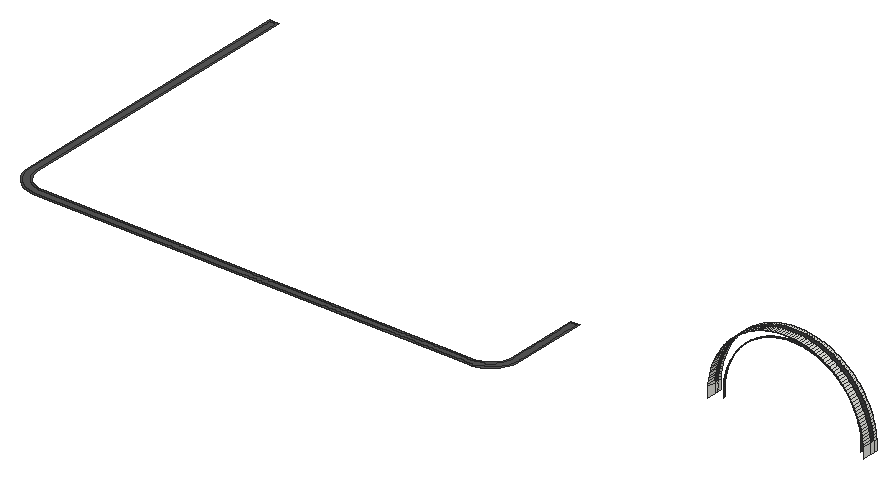
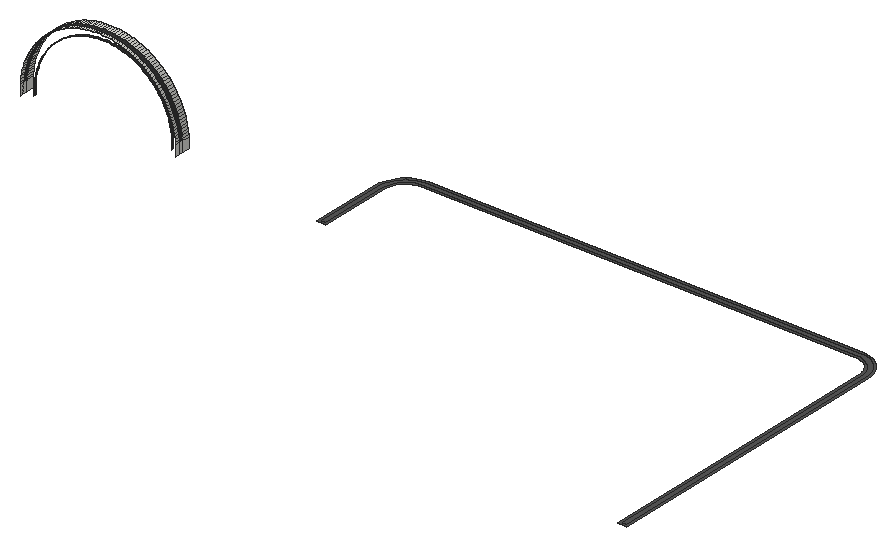
# SketchUp Ruby script. Lengths in inches.
U = 1.inch
M = Sketchup.active_model
def pt(a) = Geom::Point3d.new(a.map { |v| v * U })
def face(e, loops, mat)
  f = e.add_face(loops[0].map { |a| pt(a) })
  loops[1..].each { |l| e.add_face(l.map { |a| pt(a) }).erase! }
  f.material = f.back_material = mat if mat
  f
end
# faces: each face lists its corners as indices into pts; further lists are holes
def faces(e, pts, list, mat = nil) = list.each { |f| face(e, (f[0].is_a?(Array) ? f : [f]).map { |l| l.map { |i| pts[i] } }, mat) }
# xy, xz, yz: faces in a plane at the given z, y or x. An outline is a flat list of corners, or four numbers for a rectangle; further outlines are holes
def ring(l) = l.size == 4 ? [[l[0], l[1]], [l[2], l[1]], [l[2], l[3]], [l[0], l[3]]] : l.each_slice(2).to_a
def flat(e, list, mat, &to3) = list.each { |f| face(e, (f[0].is_a?(Array) ? f : [f]).map { |l| ring(l).map { |u, v| to3.(u, v) } }, mat) }
def xy(e, z, list, mat = nil) = flat(e, list, mat) { |x, y| [x, y, z] }
def xz(e, y, list, mat = nil) = flat(e, list, mat) { |x, z| [x, y, z] }
def yz(e, x, list, mat = nil) = flat(e, list, mat) { |y, z| [x, y, z] }
def lines(e, pts, list) = list.each { |a, b| e.add_line(pt(pts[a]), pt(pts[b])) }
# prism: a flat outline (further loops are holes) pulled along v
def prism(e, loops, v, mat = nil)
  f = face(e, loops, mat); d = Geom::Vector3d.new(v.map { |x| x * U })
  f.pushpull(f.normal.samedirection?(d) ? d.length : -d.length)
end
def box(e, o, s, mat = nil) = prism(e, [[o, [o[0] + s[0], o[1], o[2]], [o[0] + s[0], o[1] + s[1], o[2]], [o[0], o[1] + s[1], o[2]]]], [0, 0, s[2]], mat)
def at(x, y, z, deg = 0) = Geom::Transformation.translation(pt([x, y, z])) * Geom::Transformation.rotation(ORIGIN, Z_AXIS, deg.degrees)
def axes(o, x, y, z) = Geom::Transformation.new([*x, 0, *y, 0, *z, 0, *pt(o).to_a, 1])
def part(name) = M.definitions.add(name)
# library, detail: a bought-in or finely detailed component or shape, given as its bounding box
def library(name, o, s) = part(name).tap { |d| box(d.entities, o, s) }
def detail(e, o, s) = box(e.add_group.entities, o, s)
def put(e, d, t, mat = nil) = e.add_instance(d, t).tap { |i| i.material = mat if mat }
def group(e, t, mat = nil) = e.add_group.tap { |g| g.transformation = t; g.material = mat if mat }.entities
root = M.entities
M.materials.add("[Color M06]").color = [86, 86, 86]
M.materials.add("[Color M07]").color = [58, 58, 58]
xy(root,311.125,[[[45.79,42.77,294.9,42.77,296.94,42.9,299.125,43.34,301.23,44.05,303.23,45.04,304.84,46.11,305.08,46.27,306.75,47.74,308.22,49.41,308.375,49.65,309.46,51.26,310.44,53.26,311.15,55.37,311.59,57.55,311.72,59.59,311.72,102.26,306.43,102.26,306.43,59.77,306.33,58.24,306.03,56.74,305.54,55.29,304.86,53.92,304.01,52.64,303,51.49,301.85,50.48,300.58,49.63,299.2,48.95,297.75,48.46,296.25,48.16,294.72,48.0625,45.79,48.0625,44.18,48.17,42.6,48.48,41.07,49,39.63,49.71,38.29,50.61,37.08,51.67,36.01,52.88,35.12,54.22,34.41,55.67,33.89,57.19,33.57,58.77,33.47,60.38,33.47,233.58,28.18,233.58,28.18,60.38,28.33,58.08,28.78,55.82,29.52,53.64,30.53,51.57,31.81,49.66,33.33,47.93,35.07,46.41,36.98,45.13,39.05,44.11,41.23,43.37,43.49,42.92],[45.79,43.83,43.625,43.97,41.5,44.4,39.45,45.09,37.51,46.05,35.71,47.25,34.09,48.68,32.66,50.31,31.46,52.11,30.5,54.05,29.8,56.1,29.38,58.22,29.24,60.38,29.24,232.52,32.41,232.52,32.41,60.38,32.52,58.63,32.86,56.92,33.42,55.26,34.2,53.6875,35.17,52.23,36.32,50.92,37.64,49.76,39.1,48.79,40.67,48.02,42.32,47.45,44.04,47.11,45.79,47,294.72,47,296.39,47.11,298.03,47.43,299.61,47.97,301.11,48.71,302.5,49.64,303.75,50.74,304.85,52,305.78,53.38,306.52,54.88,307.06,56.47,307.38,58.1,307.49,59.77,307.49,101.2,310.66,101.2,310.66,59.625,310.53,57.6875,310.125,55.64,309.46,53.67,308.53,51.8,307.49,50.24,307.375,50.0625,306,48.49,304.43,47.12,302.69,45.96,300.82,45.04,298.85,44.37,296.8,43.96,294.87,43.83]],[45.79,43.83,294.87,43.83,296.8,43.96,298.85,44.37,300.82,45.04,302.69,45.96,304.43,47.12,306,48.49,307.375,50.0625,307.49,50.24,308.53,51.8,309.46,53.67,310.125,55.64,310.53,57.6875,310.66,59.625,310.66,101.2,307.49,101.2,307.49,59.77,307.38,58.1,307.06,56.47,306.52,54.88,305.78,53.38,304.85,52,303.75,50.74,302.5,49.64,301.11,48.71,299.61,47.97,298.03,47.43,296.39,47.11,294.72,47,45.79,47,44.04,47.11,42.32,47.45,40.67,48.02,39.1,48.79,37.64,49.76,36.32,50.92,35.17,52.23,34.2,53.6875,33.42,55.26,32.86,56.92,32.52,58.63,32.41,60.38,32.41,232.52,29.24,232.52,29.24,60.38,29.38,58.22,29.8,56.1,30.5,54.05,31.46,52.11,32.66,50.31,34.09,48.68,35.71,47.25,37.51,46.05,39.45,45.09,41.5,44.4,43.625,43.97]],"[Color M06]")
xz(root,86.25,[[398.23,311,398.23,316.97,398.22,316.88,398.15,315.41,398.13,313.94,398.15,312.47],[487.79,311,487.87,312.47,487.89,313.94,487.87,315.41,487.8,316.88,487.79,316.97]])
yz(root,398.23,[[86.25,311,90.75,316.97],[90.75,311,93.1875,316.97],[93.1875,311,95.25,316.97]])
yz(root,403.41,[[90.75,311,91.75,316.76]],"[Color M07]")
yz(root,482.61,[[90.75,311,91.75,316.76]],"[Color M07]")
yz(root,487.79,[[86.25,311,90.75,316.97],[90.75,311,93.1875,316.97],[93.1875,311,95.25,316.97]])
p = [[403.41,91.75,316.76],[403.5,91.75,317.84],[403.5,90.75,317.84],[403.41,90.75,316.76],[482.52,91.75,317.84],[482.61,91.75,316.76],
  [482.61,90.75,316.76],[482.52,90.75,317.84],[398.23,86.25,316.97],[398.23,90.75,316.97],[398.34,90.75,318.34],[398.34,86.25,318.34],
  [487.68,86.25,318.34],[487.68,90.75,318.34],[487.79,90.75,316.97],[487.79,86.25,316.97],[398.34,93.1875,318.34],[398.23,93.1875,316.97],
  [487.79,93.1875,316.97],[487.68,93.1875,318.34],[398.34,95.25,318.34],[398.23,95.25,316.97],[487.79,95.25,316.97],[487.68,95.25,318.34],
  [403.64,91.75,319.13],[403.64,90.75,319.13],[482.38,91.75,319.13],[482.38,90.75,319.13],[398.51,90.75,319.8],[398.51,86.25,319.8],
  [487.51,86.25,319.8],[487.51,90.75,319.8],[398.51,93.1875,319.8],[487.51,93.1875,319.8],[398.51,95.25,319.8],[487.51,95.25,319.8],
  [403.83,91.75,320.42],[403.83,90.75,320.42],[482.1875,91.75,320.42],[482.1875,90.75,320.42],[398.72,90.75,321.26],[398.72,86.25,321.26],
  [487.3,86.25,321.26],[487.3,90.75,321.26],[398.72,93.1875,321.26],[487.3,93.1875,321.26],[398.72,95.25,321.26],[487.3,95.25,321.26],
  [404.0625,91.75,321.7],[404.0625,90.75,321.7],[481.96,91.75,321.7],[481.96,90.75,321.7],[398.98,90.75,322.7],[398.98,86.25,322.7],
  [487.04,86.25,322.7],[487.04,90.75,322.7],[398.98,93.1875,322.7],[487.04,93.1875,322.7],[398.98,95.25,322.7],[487.04,95.25,322.7],
  [404.34,91.75,322.97],[404.34,90.75,322.97],[481.68,91.75,322.97],[481.68,90.75,322.97],[399.29,90.75,324.14],[399.29,86.25,324.14],
  [486.73,86.25,324.14],[486.73,90.75,324.14],[399.29,93.1875,324.14],[486.73,93.1875,324.14],[399.29,95.25,324.14],[486.73,95.25,324.14],
  [404.65,91.75,324.23],[404.65,90.75,324.23],[481.37,91.75,324.23],[481.37,90.75,324.23],[399.65,90.75,325.57],[399.65,86.25,325.57],
  [486.375,86.25,325.57],[486.375,90.75,325.57],[399.65,93.1875,325.57],[486.375,93.1875,325.57],[399.65,95.25,325.57],[486.375,95.25,325.57],
  [405.01,91.75,325.48],[405.01,90.75,325.48],[481.01,91.75,325.48],[481.01,90.75,325.48],[405.4,91.75,326.72],[405.4,90.75,326.72],
  [480.62,91.75,326.72],[480.62,90.75,326.72],[400.05,90.75,326.98],[400.05,86.25,326.98],[485.97,86.25,326.98],[485.97,90.75,326.98],
  [400.05,93.1875,326.98],[485.97,93.1875,326.98],[400.05,95.25,326.98],[485.97,95.25,326.98],[405.84,91.75,327.95],[405.84,90.75,327.95],
  [480.18,91.75,327.95],[480.18,90.75,327.95],[400.5,90.75,328.38],[400.5,86.25,328.38],[485.52,86.25,328.38],[485.52,90.75,328.38],
  [400.5,93.1875,328.38],[485.52,93.1875,328.38],[400.5,95.25,328.38],[485.52,95.25,328.38],[406.32,91.75,329.16],[406.32,90.75,329.16],
  [479.7,91.75,329.16],[479.7,90.75,329.16],[400.99,90.75,329.77],[400.99,86.25,329.77],[485.03,86.25,329.77],[485.03,90.75,329.77],
  [400.99,93.1875,329.77],[485.03,93.1875,329.77],[400.99,95.25,329.77],[485.03,95.25,329.77],[406.83,91.75,330.35],[406.83,90.75,330.35],
  [479.1875,91.75,330.35],[479.1875,90.75,330.35],[401.53,90.75,331.13],[401.53,86.25,331.13],[484.49,86.25,331.13],[484.49,90.75,331.13],
  [401.53,93.1875,331.13],[484.49,93.1875,331.13],[401.53,95.25,331.13],[484.49,95.25,331.13],[407.39,91.75,331.52],[407.39,90.75,331.52],
  [478.63,91.75,331.52],[478.63,90.75,331.52],[402.11,90.75,332.48],[402.11,86.25,332.48],[483.91,86.25,332.48],[483.91,90.75,332.48],
  [402.11,93.1875,332.48],[483.91,93.1875,332.48],[402.11,95.25,332.48],[483.91,95.25,332.48],[407.98,91.75,332.68],[407.98,90.75,332.68],
  [478.04,91.75,332.68],[478.04,90.75,332.68],[402.74,90.75,333.8125],[402.74,86.25,333.8125],[483.28,86.25,333.8125],[483.28,90.75,333.8125],
  [402.74,93.1875,333.8125],[483.28,93.1875,333.8125],[402.74,95.25,333.8125],[483.28,95.25,333.8125],[408.61,91.75,333.82],[408.61,90.75,333.82],
  [477.41,91.75,333.82],[477.41,90.75,333.82],[403.41,90.75,335.12],[403.41,86.25,335.12],[482.61,86.25,335.12],[482.61,90.75,335.12],
  [403.41,93.1875,335.12],[409.28,91.75,334.93],[409.28,90.75,334.93],[476.74,91.75,334.93],[476.74,90.75,334.93],[482.61,93.1875,335.12],
  [403.41,95.25,335.12],[482.61,95.25,335.12],[409.98,91.75,336.03],[409.98,90.75,336.03],[476.04,91.75,336.03],[476.04,90.75,336.03],
  [404.125,90.75,336.41],[404.125,86.25,336.41],[481.9,86.25,336.41],[481.9,90.75,336.41],[404.125,93.1875,336.41],[481.9,93.1875,336.41],
  [404.125,95.25,336.41],[481.9,95.25,336.41],[410.72,91.75,337.1],[410.72,90.75,337.1],[475.3,91.75,337.1],[475.3,90.75,337.1],
  [404.88,90.75,337.67],[404.88,86.25,337.67],[481.14,86.25,337.67],[481.14,90.75,337.67],[404.88,93.1875,337.67],[481.14,93.1875,337.67],
  [404.88,95.25,337.67],[481.14,95.25,337.67],[411.5,91.75,338.14],[411.5,90.75,338.14],[474.53,91.75,338.14],[474.53,90.75,338.14],
  [405.67,90.75,338.9],[405.67,86.25,338.9],[480.35,86.25,338.9],[480.35,90.75,338.9],[405.67,93.1875,338.9],[480.35,93.1875,338.9],
  [405.67,95.25,338.9],[480.35,95.25,338.9],[412.3,91.75,339.16],[412.3,90.75,339.16],[473.72,91.75,339.16],[473.72,90.75,339.16],
  [406.51,90.75,340.11],[406.51,86.25,340.11],[479.51,86.25,340.11],[479.51,90.75,340.11],[406.51,93.1875,340.11],[479.51,93.1875,340.11],
  [406.51,95.25,340.11],[479.51,95.25,340.11],[413.14,91.75,340.15],[413.14,90.75,340.15],[472.875,91.75,340.15],[472.875,90.75,340.15],
  [407.38,90.75,341.29],[407.38,86.25,341.29],[478.64,86.25,341.29],[478.64,90.75,341.29],[407.38,93.1875,341.29],[478.64,93.1875,341.29],
  [407.38,95.25,341.29],[478.64,95.25,341.29],[414.02,91.75,341.12],[414.02,90.75,341.12],[472,91.75,341.12],[472,90.75,341.12],
  [414.92,91.75,342.05],[414.92,90.75,342.05],[471.1,91.75,342.05],[471.1,90.75,342.05],[408.3,90.75,342.44],[408.3,86.25,342.44],
  [477.72,86.25,342.44],[477.72,90.75,342.44],[408.3,93.1875,342.44],[477.72,93.1875,342.44],[408.3,95.25,342.44],[477.72,95.25,342.44],
  [415.85,91.75,342.96],[415.85,90.75,342.96],[470.17,91.75,342.96],[470.17,90.75,342.96],[409.25,90.75,343.57],[409.25,86.25,343.57],
  [476.77,86.25,343.57],[476.77,90.75,343.57],[409.25,93.1875,343.57],[476.77,93.1875,343.57],[409.25,95.25,343.57],[476.77,95.25,343.57],
  [416.82,91.75,343.83],[416.82,90.75,343.83],[469.2,91.75,343.83],[469.2,90.75,343.83],[410.23,90.75,344.66],[410.23,86.25,344.66],
  [475.79,86.25,344.66],[475.79,90.75,344.66],[410.23,93.1875,344.66],[475.79,93.1875,344.66],[410.23,95.25,344.66],[475.79,95.25,344.66],
  [417.81,91.75,344.67],[417.81,90.75,344.67],[468.21,91.75,344.67],[468.21,90.75,344.67],[411.25,90.75,345.71],[411.25,86.25,345.71],
  [474.77,86.25,345.71],[474.77,90.75,345.71],[411.25,93.1875,345.71],[418.82,91.75,345.48],[418.82,90.75,345.48],[467.2,91.75,345.48],
  [467.2,90.75,345.48],[474.77,93.1875,345.71],[411.25,95.25,345.71],[474.77,95.25,345.71],[419.87,91.75,346.26],[419.87,90.75,346.26],
  [466.15,91.75,346.26],[466.15,90.75,346.26],[412.31,90.75,346.74],[412.31,86.25,346.74],[473.71,86.25,346.74],[473.71,90.75,346.74],
  [412.31,93.1875,346.74],[473.71,93.1875,346.74],[412.31,95.25,346.74],[473.71,95.25,346.74],[420.9375,91.75,347],[420.9375,90.75,347],
  [465.08,91.75,347],[465.08,90.75,347],[413.4,90.75,347.72],[413.4,86.25,347.72],[472.62,86.25,347.72],[472.62,90.75,347.72],
  [413.4,93.1875,347.72],[472.62,93.1875,347.72],[413.4,95.25,347.72],[472.62,95.25,347.72],[422.03,91.75,347.7],[422.03,90.75,347.7],
  [463.99,91.75,347.7],[463.99,90.75,347.7],[414.52,90.75,348.67],[414.52,86.25,348.67],[471.5,86.25,348.67],[471.5,90.75,348.67],
  [414.52,93.1875,348.67],[423.14,91.75,348.37],[423.14,90.75,348.37],[462.875,91.75,348.37],[462.875,90.75,348.37],[471.5,93.1875,348.67],
  [414.52,95.25,348.67],[471.5,95.25,348.67],[424.28,91.75,349],[424.28,90.75,349],[461.74,91.75,349],[461.74,90.75,349],
  [415.67,90.75,349.59],[415.67,86.25,349.59],[470.35,86.25,349.59],[470.35,90.75,349.59],[415.67,93.1875,349.59],[470.35,93.1875,349.59],
  [415.67,95.25,349.59],[470.35,95.25,349.59],[425.4375,91.75,349.6],[425.4375,90.75,349.6],[460.58,91.75,349.6],[460.58,90.75,349.6],
  [416.85,90.75,350.47],[416.85,86.25,350.47],[469.17,86.25,350.47],[469.17,90.75,350.47],[416.85,93.1875,350.47],[426.61,91.75,350.15],
  [426.61,90.75,350.15],[459.41,91.75,350.15],[459.41,90.75,350.15],[469.17,93.1875,350.47],[416.85,95.25,350.47],[469.17,95.25,350.47],
  [427.81,91.75,350.67],[427.81,90.75,350.67],[458.21,91.75,350.67],[458.21,90.75,350.67],[418.06,90.75,351.3],[418.06,86.25,351.3],
  [467.96,86.25,351.3],[467.96,90.75,351.3],[418.06,93.1875,351.3],[467.96,93.1875,351.3],[418.06,95.25,351.3],[467.96,95.25,351.3],
  [429.01,91.75,351.15],[429.01,90.75,351.15],[457.01,91.75,351.15],[457.01,90.75,351.15],[430.24,91.75,351.59],[430.24,90.75,351.59],
  [455.78,91.75,351.59],[455.78,90.75,351.59],[419.29,90.75,352.1],[419.29,86.25,352.1],[466.73,86.25,352.1],[466.73,90.75,352.1],
  [419.29,93.1875,352.1],[466.73,93.1875,352.1],[419.29,95.25,352.1],[466.73,95.25,352.1],[431.48,91.75,351.99],[431.48,90.75,351.99],
  [454.54,91.75,351.99],[454.54,90.75,351.99],[432.73,91.75,352.34],[432.73,90.75,352.34],[453.29,91.75,352.34],[453.29,90.75,352.34],
  [420.55,90.75,352.86],[420.55,86.25,352.86],[465.47,86.25,352.86],[465.47,90.75,352.86],[420.55,93.1875,352.86],[465.47,93.1875,352.86],
  [420.55,95.25,352.86],[465.47,95.25,352.86],[433.99,91.75,352.66],[433.99,90.75,352.66],[452.03,91.75,352.66],[452.03,90.75,352.66],
  [435.26,91.75,352.93],[435.26,90.75,352.93],[450.76,91.75,352.93],[450.76,90.75,352.93],[421.84,90.75,353.57],[421.84,86.25,353.57],
  [464.18,86.25,353.57],[464.18,90.75,353.57],[421.84,93.1875,353.57],[436.54,91.75,353.17],[436.54,90.75,353.17],[449.48,91.75,353.17],
  [449.48,90.75,353.17],[464.18,93.1875,353.57],[421.84,95.25,353.57],[464.18,95.25,353.57],[437.82,91.75,353.36],[437.82,90.75,353.36],
  [448.2,91.75,353.36],[448.2,90.75,353.36],[439.12,91.75,353.51],[439.12,90.75,353.51],[446.9,91.75,353.51],[446.9,90.75,353.51],
  [440.41,91.75,353.61],[440.41,90.75,353.61],[445.61,91.75,353.61],[445.61,90.75,353.61],[423.14,90.75,354.24],[423.14,86.25,354.24],
  [462.875,86.25,354.24],[462.875,90.75,354.24],[423.14,93.1875,354.24],[441.71,91.75,353.68],[441.71,90.75,353.68],[444.31,91.75,353.68],
  [440.73,91.75,353.61],[440.73,90.75,353.61],[444.31,90.75,353.68],[462.875,93.1875,354.24],[423.14,95.25,354.24],[462.875,95.25,354.24],
  [443.01,91.75,353.7],[443.01,90.75,353.7],[424.47,90.75,354.87],[424.47,86.25,354.87],[461.55,86.25,354.87],[461.55,90.75,354.87],
  [424.47,93.1875,354.87],[461.55,93.1875,354.87],[424.47,95.25,354.87],[461.55,95.25,354.87],[425.82,90.75,355.46],[425.82,86.25,355.46],
  [460.2,86.25,355.46],[460.2,90.75,355.46],[425.82,93.1875,355.46],[460.2,93.1875,355.46],[425.82,95.25,355.46],[460.2,95.25,355.46],
  [427.1875,90.75,356],[427.1875,86.25,356],[458.83,86.25,356],[458.83,90.75,356],[427.1875,93.1875,356],[458.83,93.1875,356],
  [427.1875,95.25,356],[458.83,95.25,356],[428.57,90.75,356.49],[428.57,86.25,356.49],[457.45,86.25,356.49],[457.45,90.75,356.49],
  [428.57,93.1875,356.49],[457.45,93.1875,356.49],[428.57,95.25,356.49],[457.45,95.25,356.49],[429.97,90.75,356.94],[429.97,86.25,356.94],
  [456.05,86.25,356.94],[456.05,90.75,356.94],[429.97,93.1875,356.94],[456.05,93.1875,356.94],[429.97,95.25,356.94],[456.05,95.25,356.94],
  [431.38,90.75,357.35],[431.38,86.25,357.35],[454.64,86.25,357.35],[454.64,90.75,357.35],[431.38,93.1875,357.35],[454.64,93.1875,357.35],
  [431.38,95.25,357.35],[454.64,95.25,357.35],[432.8125,90.75,357.7],[432.8125,86.25,357.7],[453.21,86.25,357.7],[453.21,90.75,357.7],
  [432.8125,93.1875,357.7],[453.21,93.1875,357.7],[432.8125,95.25,357.7],[453.21,95.25,357.7],[434.25,90.75,358.01],[434.25,86.25,358.01],
  [451.77,86.25,358.01],[451.77,90.75,358.01],[434.25,93.1875,358.01],[451.77,93.1875,358.01],[434.25,95.25,358.01],[451.77,95.25,358.01],
  [435.69,90.75,358.28],[435.69,86.25,358.28],[450.33,86.25,358.28],[450.33,90.75,358.28],[435.69,93.1875,358.28],[450.33,93.1875,358.28],
  [435.69,95.25,358.28],[450.33,95.25,358.28],[437.15,90.75,358.49],[437.15,86.25,358.49],[448.87,86.25,358.49],[448.87,90.75,358.49],
  [437.15,93.1875,358.49],[448.87,93.1875,358.49],[437.15,95.25,358.49],[448.87,95.25,358.49],[438.61,90.75,358.66],[438.61,86.25,358.66],
  [447.41,86.25,358.66],[447.41,90.75,358.66],[438.61,93.1875,358.66],[447.41,93.1875,358.66],[438.61,95.25,358.66],[447.41,95.25,358.66],
  [440.07,90.75,358.78],[440.07,86.25,358.78],[445.95,86.25,358.78],[445.95,90.75,358.78],[440.07,93.1875,358.78],[445.95,93.1875,358.78],
  [440.07,95.25,358.78],[445.95,95.25,358.78],[441.54,90.75,358.85],[441.54,86.25,358.85],[444.48,86.25,358.85],[444.48,90.75,358.85],
  [441.54,93.1875,358.85],[444.48,93.1875,358.85],[441.54,95.25,358.85],[444.48,95.25,358.85],[443.01,90.75,358.88],[443.01,86.25,358.88],
  [443.01,93.1875,358.88],[443.01,95.25,358.88]]
faces(root,p,[[0,1,2,3],[4,5,6,7],[16,17,9,10],[18,19,13,14],[1,24,25,2],[26,4,7,27],[32,16,10,28],[19,33,31,13],
  [24,36,37,25],[38,26,27,39],[44,32,28,40],[33,45,43,31],[36,48,49,37],[50,38,39,51],[56,44,40,52],[45,57,55,43],
  [48,60,61,49],[62,50,51,63],[68,56,52,64],[57,69,67,55],[60,72,73,61],[74,62,63,75],[80,68,64,76],[69,81,79,67],
  [72,84,85,73],[86,74,75,87],[84,88,89,85],[90,86,87,91],[96,80,76,92],[81,97,95,79],[88,100,101,89],[102,90,91,103],
  [108,96,92,104],[97,109,107,95],[100,112,113,101],[114,102,103,115],[120,108,104,116],[109,121,119,107],[112,124,125,113],[126,114,115,127],
  [132,120,116,128],[121,133,131,119],[124,136,137,125],[138,126,127,139],[144,132,128,140],[133,145,143,131],[136,148,149,137],[150,138,139,151],
  [156,144,140,152],[145,157,155,143],[148,160,161,149],[162,150,151,163],[168,156,152,164],[160,169,170,161],[171,162,163,172],[157,173,167,155],
  [169,176,177,170],[178,171,172,179],[184,168,164,180],[173,185,183,167],[176,188,189,177],[190,178,179,191],[196,184,180,192],[185,197,195,183],
  [188,200,201,189],[202,190,191,203],[208,196,192,204],[197,209,207,195],[200,212,213,201],[214,202,203,215],[220,208,204,216],[209,221,219,207],
  [212,224,225,213],[226,214,215,227],[232,220,216,228],[221,233,231,219],[224,236,237,225],[238,226,227,239],[236,240,241,237],[242,238,239,243],
  [248,232,228,244],[233,249,247,231],[240,252,253,241],[254,242,243,255],[260,248,244,256],[249,261,259,247],[252,264,265,253],[266,254,255,267],
  [272,260,256,268],[261,273,271,259],[264,276,277,265],[278,266,267,279],[284,272,268,280],[276,285,286,277],[287,278,279,288],[273,289,283,271],
  [285,292,293,286],[294,287,288,295],[300,284,280,296],[289,301,299,283],[292,304,305,293],[306,294,295,307],[312,300,296,308],[301,313,311,299],
  [304,316,317,305],[318,306,307,319],[324,312,308,320],[316,325,326,317],[327,318,319,328],[313,329,323,311],[325,332,333,326],[334,327,328,335],
  [340,324,320,336],[329,341,339,323],[332,344,345,333],[346,334,335,347],[352,340,336,348],[344,353,354,345],[355,346,347,356],[341,357,351,339],
  [353,360,361,354],[362,355,356,363],[368,352,348,364],[357,369,367,351],[360,372,373,361],[374,362,363,375],[372,376,377,373],[378,374,375,379],
  [384,368,364,380],[369,385,383,367],[376,388,389,377],[390,378,379,391],[388,392,393,389],[394,390,391,395],[400,384,380,396],[385,401,399,383],
  [392,404,405,393],[406,394,395,407],[404,408,409,405],[410,406,407,411],[416,400,396,412],[408,417,418,409],[419,410,411,420],[401,421,415,399],
  [417,424,425,418],[426,419,420,427],[424,428,429,425],[430,426,427,431],[428,432,433,429],[434,430,431,435],[440,416,412,436],[432,441,442,433],
  [443,434,435,446],[421,447,439,415],[441,450,451,442],[450,443,446,451],[456,440,436,452],[447,457,455,439],[464,456,452,460],[457,465,463,455],
  [472,464,460,468],[465,473,471,463],[480,472,468,476],[473,481,479,471],[488,480,476,484],[481,489,487,479],[496,488,484,492],[489,497,495,487],
  [504,496,492,500],[497,505,503,495],[512,504,500,508],[505,513,511,503],[520,512,508,516],[513,521,519,511],[528,520,516,524],[521,529,527,519],
  [536,528,524,532],[529,537,535,527],[544,536,532,540],[537,545,543,535],[552,544,540,548],[545,553,551,543],[558,552,548,556],[553,558,556,551]],"[Color M07]")
faces(root,p,[[8,9,10,11],[12,13,14,15],[20,16,17,21],[22,18,19,23],[11,10,28,29],[30,31,13,12],[34,32,16,20],[23,19,33,35],
  [29,28,40,41],[42,43,31,30],[46,44,32,34],[35,33,45,47],[41,40,52,53],[54,55,43,42],[58,56,44,46],[47,45,57,59],
  [53,52,64,65],[66,67,55,54],[70,68,56,58],[59,57,69,71],[65,64,76,77],[78,79,67,66],[82,80,68,70],[71,69,81,83],
  [77,76,92,93],[94,95,79,78],[98,96,80,82],[83,81,97,99],[93,92,104,105],[106,107,95,94],[110,108,96,98],[99,97,109,111],
  [105,104,116,117],[118,119,107,106],[122,120,108,110],[111,109,121,123],[117,116,128,129],[130,131,119,118],[134,132,120,122],[123,121,133,135],
  [129,128,140,141],[142,143,131,130],[146,144,132,134],[135,133,145,147],[141,140,152,153],[154,155,143,142],[158,156,144,146],[147,145,157,159],
  [153,152,164,165],[166,167,155,154],[174,168,156,158],[159,157,173,175],[165,164,180,181],[182,183,167,166],[186,184,168,174],[175,173,185,187],
  [181,180,192,193],[194,195,183,182],[198,196,184,186],[187,185,197,199],[193,192,204,205],[206,207,195,194],[210,208,196,198],[199,197,209,211],
  [205,204,216,217],[218,219,207,206],[222,220,208,210],[211,209,221,223],[217,216,228,229],[230,231,219,218],[234,232,220,222],[223,221,233,235],
  [229,228,244,245],[246,247,231,230],[250,248,232,234],[235,233,249,251],[245,244,256,257],[258,259,247,246],[262,260,248,250],[251,249,261,263],
  [257,256,268,269],[270,271,259,258],[274,272,260,262],[263,261,273,275],[269,268,280,281],[282,283,271,270],[290,284,272,274],[275,273,289,291],
  [281,280,296,297],[298,299,283,282],[302,300,284,290],[291,289,301,303],[297,296,308,309],[310,311,299,298],[314,312,300,302],[303,301,313,315],
  [309,308,320,321],[322,323,311,310],[330,324,312,314],[315,313,329,331],[321,320,336,337],[338,339,323,322],[342,340,324,330],[331,329,341,343],
  [337,336,348,349],[350,351,339,338],[358,352,340,342],[343,341,357,359],[349,348,364,365],[366,367,351,350],[370,368,352,358],[359,357,369,371],
  [365,364,380,381],[382,383,367,366],[386,384,368,370],[371,369,385,387],[381,380,396,397],[398,399,383,382],[402,400,384,386],[387,385,401,403],
  [397,396,412,413],[414,415,399,398],[422,416,400,402],[403,401,421,423],[413,412,436,437],[438,439,415,414],[443,444,445,446],[448,440,416,422],
  [423,421,447,449],[437,436,452,453],[454,455,439,438],[458,456,440,448],[449,447,457,459],[453,452,460,461],[462,463,455,454],[466,464,456,458],
  [459,457,465,467],[461,460,468,469],[470,471,463,462],[474,472,464,466],[467,465,473,475],[469,468,476,477],[478,479,471,470],[482,480,472,474],
  [475,473,481,483],[477,476,484,485],[486,487,479,478],[490,488,480,482],[483,481,489,491],[485,484,492,493],[494,495,487,486],[498,496,488,490],
  [491,489,497,499],[493,492,500,501],[502,503,495,494],[506,504,496,498],[499,497,505,507],[501,500,508,509],[510,511,503,502],[514,512,504,506],
  [507,505,513,515],[509,508,516,517],[518,519,511,510],[522,520,512,514],[515,513,521,523],[517,516,524,525],[526,527,519,518],[530,528,520,522],
  [523,521,529,531],[525,524,532,533],[534,535,527,526],[538,536,528,530],[531,529,537,539],[533,532,540,541],[542,543,535,534],[546,544,536,538],
  [539,537,545,547],[541,540,548,549],[550,551,543,542],[554,552,544,546],[547,545,553,555],[549,548,556,557],[557,556,551,550],[559,558,552,554],
  [555,553,558,559]])
